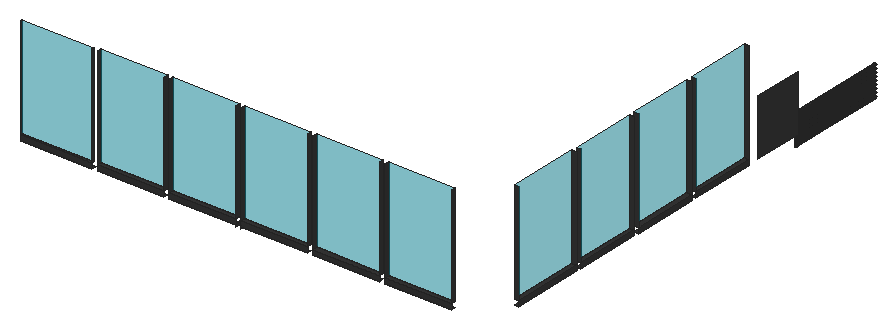
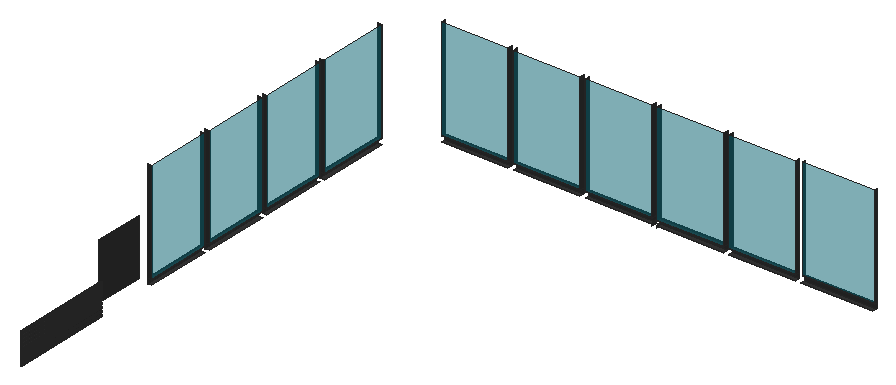
# SketchUp Ruby script. Lengths in inches.
U = 1.inch
M = Sketchup.active_model
def pt(a) = Geom::Point3d.new(a.map { |v| v * U })
def face(e, loops, mat)
  f = e.add_face(loops[0].map { |a| pt(a) })
  loops[1..].each { |l| e.add_face(l.map { |a| pt(a) }).erase! }
  f.material = f.back_material = mat if mat
  f
end
# faces: each face lists its corners as indices into pts; further lists are holes
def faces(e, pts, list, mat = nil) = list.each { |f| face(e, (f[0].is_a?(Array) ? f : [f]).map { |l| l.map { |i| pts[i] } }, mat) }
# xy, xz, yz: faces in a plane at the given z, y or x. An outline is a flat list of corners, or four numbers for a rectangle; further outlines are holes
def ring(l) = l.size == 4 ? [[l[0], l[1]], [l[2], l[1]], [l[2], l[3]], [l[0], l[3]]] : l.each_slice(2).to_a
def flat(e, list, mat, &to3) = list.each { |f| face(e, (f[0].is_a?(Array) ? f : [f]).map { |l| ring(l).map { |u, v| to3.(u, v) } }, mat) }
def xy(e, z, list, mat = nil) = flat(e, list, mat) { |x, y| [x, y, z] }
def xz(e, y, list, mat = nil) = flat(e, list, mat) { |x, z| [x, y, z] }
def yz(e, x, list, mat = nil) = flat(e, list, mat) { |y, z| [x, y, z] }
def lines(e, pts, list) = list.each { |a, b| e.add_line(pt(pts[a]), pt(pts[b])) }
# prism: a flat outline (further loops are holes) pulled along v
def prism(e, loops, v, mat = nil)
  f = face(e, loops, mat); d = Geom::Vector3d.new(v.map { |x| x * U })
  f.pushpull(f.normal.samedirection?(d) ? d.length : -d.length)
end
def box(e, o, s, mat = nil) = prism(e, [[o, [o[0] + s[0], o[1], o[2]], [o[0] + s[0], o[1] + s[1], o[2]], [o[0], o[1] + s[1], o[2]]]], [0, 0, s[2]], mat)
def at(x, y, z, deg = 0) = Geom::Transformation.translation(pt([x, y, z])) * Geom::Transformation.rotation(ORIGIN, Z_AXIS, deg.degrees)
def axes(o, x, y, z) = Geom::Transformation.new([*x, 0, *y, 0, *z, 0, *pt(o).to_a, 1])
def part(name) = M.definitions.add(name)
# library, detail: a bought-in or finely detailed component or shape, given as its bounding box
def library(name, o, s) = part(name).tap { |d| box(d.entities, o, s) }
def detail(e, o, s) = box(e.add_group.entities, o, s)
def put(e, d, t, mat = nil) = e.add_instance(d, t).tap { |i| i.material = mat if mat }
def group(e, t, mat = nil) = e.add_group.tap { |g| g.transformation = t; g.material = mat if mat }.entities
root = M.entities
M.materials.add("[0135_DarkGray]1").color = [53, 53, 53]
M.materials.add("[Translucent Glass Blue]1").color = [1, 149, 171]
M.materials["[Translucent Glass Blue]1"].alpha = 0.5
xy(root,442.86,[[1035.97,1165.35,1036.3125,1278.6875]],"[0135_DarkGray]1")
xy(root,445.46,[[1035.96,1165.35,1036.3,1278.6875]],"[0135_DarkGray]1")
xy(root,446.99,[[1035.97,1165.35,1036.3125,1278.6875]],"[0135_DarkGray]1")
xy(root,450.375,[[497.69,732.5625,579.69,737.5625],[585.69,732.5625,661.69,737.5625],[667.69,732.5625,743.69,737.5625],[749.69,732.5625,825.69,737.5625],[831.69,732.5625,907.69,737.5625],
  [913.69,732.5625,989.69,737.5625],[1028.13,774.6875,1033.13,856.6875],[1028.13,862.6875,1033.13,938.6875],[1028.13,944.6875,1033.13,1020.6875],[1028.13,1026.6875,1033.13,1102.6875]],"[0135_DarkGray]1")
xy(root,451.125,[[1035.97,1165.35,1036.3125,1278.6875]],"[0135_DarkGray]1")
xy(root,453.73,[[1035.96,1165.35,1036.3,1278.6875]],"[0135_DarkGray]1")
xy(root,455.26,[[1035.97,1165.35,1036.3125,1278.6875]],"[0135_DarkGray]1")
xy(root,456.375,[[497.69,732.5625,579.69,734.5625],[585.69,732.5625,661.69,737.5625],[667.69,732.5625,743.69,737.5625],[749.69,732.5625,825.69,737.5625],[831.69,732.5625,907.69,737.5625],
  [913.69,732.5625,989.69,737.5625],[1028.13,774.6875,1033.13,856.6875],[1028.13,862.6875,1033.13,938.6875],[1028.13,944.6875,1033.13,1020.6875],[1028.13,1026.6875,1033.13,1102.6875]],"[0135_DarkGray]1")
xy(root,457.86,[[1035.96,1165.35,1036.3,1278.6875]],"[0135_DarkGray]1")
xy(root,459.39,[[1035.97,1165.35,1036.3125,1278.6875]],"[0135_DarkGray]1")
xy(root,467.66,[[1035.97,1165.35,1036.3125,1278.6875]],"[0135_DarkGray]1")
xy(root,470.26,[[1035.96,1165.35,1036.3,1278.6875]],"[0135_DarkGray]1")
xy(root,471.79,[[1035.97,1165.35,1036.3125,1278.6875]],"[0135_DarkGray]1")
xy(root,478.53,[[1035.96,1165.35,1036.3,1278.6875]],"[0135_DarkGray]1")
xz(root,732.5625,[[497.69,450.375,579.69,456.375],[585.69,450.375,661.69,456.375],[667.69,450.375,743.69,456.375],[749.69,450.375,825.69,456.375],[831.69,450.375,907.69,456.375],
  [913.69,450.375,989.69,456.375]],"[0135_DarkGray]1")
xz(root,734.5625,[[497.69,456.375,579.69,572.5]],"[Translucent Glass Blue]1")
xz(root,737.5625,[[585.69,456.375,661.69,572.5],[667.69,456.375,743.69,572.5],[749.69,456.375,825.69,572.5],[831.69,456.375,907.69,572.5],[913.69,456.375,989.69,572.5]],"[Translucent Glass Blue]1")
xz(root,774.6875,[[1028.13,456.375,1033.13,572.5]],"[0135_DarkGray]1")
xz(root,856.6875,[[1028.13,456.375,1033.13,572.5]],"[0135_DarkGray]1")
xz(root,862.6875,[[1028.13,456.375,1033.13,572.5]],"[0135_DarkGray]1")
xz(root,938.6875,[[1028.13,456.375,1033.13,572.5]],"[0135_DarkGray]1")
xz(root,944.6875,[[1028.13,456.375,1033.13,572.5]],"[0135_DarkGray]1")
xz(root,1020.6875,[[1028.13,456.375,1033.13,572.5]],"[0135_DarkGray]1")
xz(root,1026.6875,[[1028.13,456.375,1033.13,572.5]],"[0135_DarkGray]1")
xz(root,1102.6875,[[1028.13,456.375,1033.13,572.5]],"[0135_DarkGray]1")
yz(root,497.69,[[732.5625,456.375,734.5625,572.5]],"[0135_DarkGray]1")
yz(root,579.69,[[732.5625,456.375,734.5625,572.5]],"[0135_DarkGray]1")
yz(root,585.69,[[732.5625,456.375,737.5625,572.5]],"[0135_DarkGray]1")
yz(root,661.69,[[732.5625,456.375,737.5625,572.5]],"[0135_DarkGray]1")
yz(root,667.69,[[732.5625,456.375,737.5625,572.5]],"[0135_DarkGray]1")
yz(root,743.69,[[732.5625,448.5,737.5625,450.375],[732.5625,456.375,737.5625,456.77],[732.5625,456.77,737.5625,572.5]],"[0135_DarkGray]1")
yz(root,749.69,[[732.5625,448.5,737.5625,450.375],[732.5625,456.375,737.5625,456.77],[732.5625,456.77,737.5625,572.5]],"[0135_DarkGray]1")
yz(root,825.69,[[732.5625,456.375,737.5625,572.5]],"[0135_DarkGray]1")
yz(root,831.69,[[732.5625,456.375,737.5625,572.5]],"[0135_DarkGray]1")
yz(root,907.69,[[732.5625,456.375,737.5625,572.5]],"[0135_DarkGray]1")
yz(root,913.69,[[732.5625,456.375,737.5625,572.5]],"[0135_DarkGray]1")
yz(root,989.69,[[732.5625,456.375,737.5625,572.5]],"[0135_DarkGray]1")
yz(root,1028.13,[[774.6875,456.375,856.6875,572.5],[862.6875,456.375,938.6875,572.5],[944.6875,456.375,1020.6875,572.5],[1026.6875,456.375,1102.6875,572.5]],"[Translucent Glass Blue]1")
yz(root,1033.13,[[774.6875,450.375,856.6875,456.375],[862.6875,450.375,938.6875,456.375],[944.6875,450.375,1020.6875,456.375],[1026.6875,450.375,1102.6875,456.375]],"[0135_DarkGray]1")
yz(root,1034.83,[[1165.35,443.98,1278.6875,444.32],[1165.35,448.11,1278.6875,448.46],[1165.35,452.25,1278.6875,452.59],[1165.35,456.38,1278.6875,456.72],[1165.35,460.51,1278.6875,460.86],
  [1165.35,464.65,1278.6875,464.99],[1165.35,468.78,1278.6875,469.125],[1165.35,472.91,1278.6875,473.26],[1165.35,477.05,1278.6875,477.39]],"[0135_DarkGray]1")
yz(root,1038.13,[[1108.6875,456.375,1165.35,520.4375]],"[0135_DarkGray]1")
p = [[1035.64,1165.35,442.94],[1035.34,1165.35,443.11],[1035.34,1278.6875,443.11],[1035.64,1278.6875,442.94],[1035.97,1165.35,442.86],[1035.97,1278.6875,442.86],
  [1036.64,1165.35,442.95],[1036.3125,1165.35,442.86],[1036.3125,1278.6875,442.86],[1036.64,1278.6875,442.95],[1036.94,1165.35,443.12],[1036.94,1278.6875,443.12],
  [1035.1,1165.35,443.35],[1035.1,1278.6875,443.35],[1037.18,1165.35,443.37],[1037.18,1278.6875,443.37],[1034.93,1165.35,443.65],[1034.93,1278.6875,443.65],
  [1037.35,1165.35,443.66],[1037.35,1278.6875,443.66],[1034.83,1165.35,443.98],[1034.83,1278.6875,443.98],[1037.4375,1165.35,444],[1037.4375,1278.6875,444],
  [1037.44,1165.35,444.34],[1037.44,1278.6875,444.34],[1034.83,1165.35,444.32],[1034.92,1165.35,444.65],[1034.92,1278.6875,444.65],[1034.83,1278.6875,444.32],
  [1037.34,1165.35,444.67],[1037.34,1278.6875,444.67],[1035.09,1165.35,444.95],[1035.09,1278.6875,444.95],[1037.17,1165.35,444.96],[1037.17,1278.6875,444.96],
  [1035.33,1165.35,445.2],[1035.33,1278.6875,445.2],[1036.93,1165.35,445.21],[1036.93,1278.6875,445.21],[1035.625,1165.35,445.37],[1035.625,1278.6875,445.37],
  [1036.63,1165.35,445.375],[1036.63,1278.6875,445.375],[1035.96,1165.35,445.46],[1035.96,1278.6875,445.46],[1036.3,1165.35,445.46],[1036.3,1278.6875,445.46],
  [1035.97,1165.35,446.99],[1035.64,1165.35,447.08],[1035.64,1278.6875,447.08],[1035.97,1278.6875,446.99],[1036.64,1165.35,447.08],[1036.3125,1165.35,446.99],
  [1036.3125,1278.6875,446.99],[1036.64,1278.6875,447.08],[1035.34,1165.35,447.25],[1035.34,1278.6875,447.25],[1036.94,1165.35,447.26],[1036.94,1278.6875,447.26],
  [1035.1,1165.35,447.49],[1035.1,1278.6875,447.49],[1037.18,1165.35,447.5],[1037.18,1278.6875,447.5],[1034.93,1165.35,447.78],[1034.93,1278.6875,447.78],
  [1037.35,1165.35,447.8],[1037.35,1278.6875,447.8],[1034.83,1165.35,448.11],[1034.83,1278.6875,448.11],[1037.4375,1165.35,448.13],[1037.4375,1278.6875,448.13],
  [1037.44,1165.35,448.47],[1037.44,1278.6875,448.47],[1034.83,1165.35,448.46],[1034.92,1165.35,448.79],[1034.92,1278.6875,448.79],[1034.83,1278.6875,448.46],
  [1037.34,1165.35,448.8],[1037.34,1278.6875,448.8],[1035.09,1165.35,449.09],[1035.09,1278.6875,449.09],[1037.17,1165.35,449.1],[1037.17,1278.6875,449.1],
  [1035.33,1165.35,449.33],[1035.33,1278.6875,449.33],[1036.93,1165.35,449.34],[1036.93,1278.6875,449.34],[1035.625,1165.35,449.5],[1035.625,1278.6875,449.5],
  [1036.63,1165.35,449.51],[1036.63,1278.6875,449.51],[1035.96,1165.35,449.59],[1035.96,1278.6875,449.59],[1036.3,1165.35,449.6],[1036.3,1278.6875,449.6],
  [1035.97,1165.35,451.125],[1035.64,1165.35,451.21],[1035.64,1278.6875,451.21],[1035.97,1278.6875,451.125],[1036.64,1165.35,451.22],[1036.3125,1165.35,451.125],
  [1036.3125,1278.6875,451.125],[1036.64,1278.6875,451.22],[1035.34,1165.35,451.38],[1035.34,1278.6875,451.38],[1036.94,1165.35,451.39],[1036.94,1278.6875,451.39],
  [1035.1,1165.35,451.62],[1035.1,1278.6875,451.62],[1037.18,1165.35,451.63],[1037.18,1278.6875,451.63],[1034.93,1165.35,451.92],[1034.93,1278.6875,451.92],
  [1037.35,1165.35,451.93],[1037.35,1278.6875,451.93],[1034.83,1165.35,452.25],[1034.83,1278.6875,452.25],[1037.4375,1165.35,452.26],[1037.4375,1278.6875,452.26],
  [1037.44,1165.35,452.6],[1037.44,1278.6875,452.6],[1034.83,1165.35,452.59],[1034.92,1165.35,452.92],[1034.92,1278.6875,452.92],[1034.83,1278.6875,452.59],
  [1037.34,1165.35,452.94],[1037.34,1278.6875,452.94],[1035.09,1165.35,453.22],[1035.09,1278.6875,453.22],[1037.17,1165.35,453.23],[1037.17,1278.6875,453.23],
  [1035.33,1165.35,453.46],[1035.33,1278.6875,453.46],[1036.93,1165.35,453.47],[1036.93,1278.6875,453.47],[1035.625,1165.35,453.64],[1035.625,1278.6875,453.64],
  [1036.63,1165.35,453.64],[1036.63,1278.6875,453.64],[1035.96,1165.35,453.73],[1035.96,1278.6875,453.73],[1036.3,1165.35,453.73],[1036.3,1278.6875,453.73],
  [1035.64,1165.35,455.34],[1035.34,1165.35,455.51],[1035.34,1278.6875,455.51],[1035.64,1278.6875,455.34],[1035.97,1165.35,455.26],[1035.97,1278.6875,455.26],
  [1036.64,1165.35,455.35],[1036.3125,1165.35,455.26],[1036.3125,1278.6875,455.26],[1036.64,1278.6875,455.35],[1036.94,1165.35,455.52],[1036.94,1278.6875,455.52],
  [1035.1,1165.35,455.75],[1035.1,1278.6875,455.75],[1037.18,1165.35,455.77],[1037.18,1278.6875,455.77],[1034.93,1165.35,456.05],[1034.93,1278.6875,456.05],
  [1037.35,1165.35,456.0625],[1037.35,1278.6875,456.0625],[1034.83,1165.35,456.38],[1034.83,1278.6875,456.38],[1037.4375,1165.35,456.4],[1037.4375,1278.6875,456.4],
  [1037.44,1165.35,456.74],[1037.44,1278.6875,456.74],[1034.83,1165.35,456.72],[1034.92,1165.35,457.05],[1034.92,1278.6875,457.05],[1034.83,1278.6875,456.72],
  [1037.34,1165.35,457.07],[1037.34,1278.6875,457.07],[1035.09,1165.35,457.35],[1035.09,1278.6875,457.35],[1037.17,1165.35,457.36],[1037.17,1278.6875,457.36],
  [1035.33,1165.35,457.6],[1035.33,1278.6875,457.6],[1036.93,1165.35,457.61],[1036.93,1278.6875,457.61],[1035.625,1165.35,457.77],[1035.625,1278.6875,457.77],
  [1036.63,1165.35,457.77],[1036.63,1278.6875,457.77],[1035.96,1165.35,457.86],[1035.96,1278.6875,457.86],[1036.3,1165.35,457.86],[1036.3,1278.6875,457.86],
  [1035.97,1165.35,459.39],[1035.64,1165.35,459.48],[1035.64,1278.6875,459.48],[1035.97,1278.6875,459.39],[1036.64,1165.35,459.48],[1036.3125,1165.35,459.39],
  [1036.3125,1278.6875,459.39],[1036.64,1278.6875,459.48],[1035.34,1165.35,459.65],[1035.34,1278.6875,459.65],[1036.94,1165.35,459.66],[1036.94,1278.6875,459.66],
  [1035.1,1165.35,459.89],[1035.1,1278.6875,459.89],[1037.18,1165.35,459.9],[1037.18,1278.6875,459.9],[1034.93,1165.35,460.18],[1034.93,1278.6875,460.18],
  [1037.35,1165.35,460.2],[1037.35,1278.6875,460.2],[1034.83,1165.35,460.51],[1034.83,1278.6875,460.51],[1037.4375,1165.35,460.53],[1037.4375,1278.6875,460.53],
  [1037.44,1165.35,460.87],[1037.44,1278.6875,460.87],[1034.83,1165.35,460.86],[1034.92,1165.35,461.1875],[1034.92,1278.6875,461.1875],[1034.83,1278.6875,460.86],
  [1037.34,1165.35,461.2],[1037.34,1278.6875,461.2],[1035.09,1165.35,461.49],[1035.09,1278.6875,461.49],[1037.17,1165.35,461.5],[1037.17,1278.6875,461.5],
  [1035.33,1165.35,461.73],[1035.33,1278.6875,461.73],[1036.93,1165.35,461.74],[1036.93,1278.6875,461.74],[1035.625,1165.35,461.9],[1035.625,1278.6875,461.9],
  [1036.63,1165.35,461.91],[1036.63,1278.6875,461.91],[1035.96,1165.35,461.99],[1035.96,1278.6875,461.99],[1036.3,1165.35,462],[1036.3,1278.6875,462],
  [1035.97,1165.35,463.52],[1035.64,1165.35,463.61],[1035.64,1278.6875,463.61],[1035.97,1278.6875,463.52],[1036.3125,1165.35,463.53],[1036.3125,1278.6875,463.53],
  [1036.64,1165.35,463.62],[1036.64,1278.6875,463.62],[1035.34,1165.35,463.78],[1035.34,1278.6875,463.78],[1036.94,1165.35,463.79],[1036.94,1278.6875,463.79],
  [1035.1,1165.35,464.02],[1035.1,1278.6875,464.02],[1037.18,1165.35,464.03],[1037.18,1278.6875,464.03],[1034.93,1165.35,464.32],[1034.93,1278.6875,464.32],
  [1037.35,1165.35,464.33],[1037.35,1278.6875,464.33],[1034.83,1165.35,464.65],[1034.83,1278.6875,464.65],[1037.4375,1165.35,464.66],[1037.4375,1278.6875,464.66],
  [1037.44,1165.35,465],[1037.44,1278.6875,465],[1034.83,1165.35,464.99],[1034.92,1165.35,465.32],[1034.92,1278.6875,465.32],[1034.83,1278.6875,464.99],
  [1037.34,1165.35,465.34],[1037.34,1278.6875,465.34],[1035.09,1165.35,465.62],[1035.09,1278.6875,465.62],[1037.17,1165.35,465.63],[1037.17,1278.6875,465.63],
  [1035.33,1165.35,465.86],[1035.33,1278.6875,465.86],[1036.93,1165.35,465.87],[1036.93,1278.6875,465.87],[1035.625,1165.35,466.04],[1035.625,1278.6875,466.04],
  [1036.63,1165.35,466.04],[1036.63,1278.6875,466.04],[1035.96,1165.35,466.125],[1035.96,1278.6875,466.125],[1036.3,1165.35,466.13],[1036.3,1278.6875,466.13],
  [1035.64,1165.35,467.74],[1035.34,1165.35,467.91],[1035.34,1278.6875,467.91],[1035.64,1278.6875,467.74],[1035.97,1165.35,467.66],[1035.97,1278.6875,467.66],
  [1036.64,1165.35,467.75],[1036.3125,1165.35,467.66],[1036.3125,1278.6875,467.66],[1036.64,1278.6875,467.75],[1036.94,1165.35,467.92],[1036.94,1278.6875,467.92],
  [1035.1,1165.35,468.15],[1035.1,1278.6875,468.15],[1037.18,1165.35,468.17],[1037.18,1278.6875,468.17],[1034.93,1165.35,468.45],[1034.93,1278.6875,468.45],
  [1037.35,1165.35,468.46],[1037.35,1278.6875,468.46],[1034.83,1165.35,468.78],[1034.83,1278.6875,468.78],[1037.4375,1165.35,468.8],[1037.4375,1278.6875,468.8],
  [1037.44,1165.35,469.14],[1037.44,1278.6875,469.14],[1034.83,1165.35,469.125],[1034.92,1165.35,469.45],[1034.92,1278.6875,469.45],[1034.83,1278.6875,469.125],
  [1037.34,1165.35,469.47],[1037.34,1278.6875,469.47],[1035.09,1165.35,469.75],[1035.09,1278.6875,469.75],[1037.17,1165.35,469.76],[1037.17,1278.6875,469.76],
  [1035.33,1165.35,470],[1035.33,1278.6875,470],[1036.93,1165.35,470.01],[1036.93,1278.6875,470.01],[1035.625,1165.35,470.17],[1035.625,1278.6875,470.17],
  [1036.63,1165.35,470.17],[1036.63,1278.6875,470.17],[1035.96,1165.35,470.26],[1035.96,1278.6875,470.26],[1036.3,1165.35,470.26],[1036.3,1278.6875,470.26],
  [1035.97,1165.35,471.79],[1035.64,1165.35,471.88],[1035.64,1278.6875,471.88],[1035.97,1278.6875,471.79],[1036.64,1165.35,471.88],[1036.3125,1165.35,471.79],
  [1036.3125,1278.6875,471.79],[1036.64,1278.6875,471.88],[1035.34,1165.35,472.05],[1035.34,1278.6875,472.05],[1036.94,1165.35,472.06],[1036.94,1278.6875,472.06],
  [1035.1,1165.35,472.29],[1035.1,1278.6875,472.29],[1037.18,1165.35,472.3],[1037.18,1278.6875,472.3],[1034.93,1165.35,472.58],[1034.93,1278.6875,472.58],
  [1037.35,1165.35,472.6],[1037.35,1278.6875,472.6],[1034.83,1165.35,472.91],[1034.83,1278.6875,472.91],[1037.4375,1165.35,472.93],[1037.4375,1278.6875,472.93],
  [1037.44,1165.35,473.27],[1037.44,1278.6875,473.27],[1034.83,1165.35,473.26],[1034.92,1165.35,473.59],[1034.92,1278.6875,473.59],[1034.83,1278.6875,473.26],
  [1037.34,1165.35,473.6],[1037.34,1278.6875,473.6],[1035.09,1165.35,473.89],[1035.09,1278.6875,473.89],[1037.17,1165.35,473.9],[1037.17,1278.6875,473.9],
  [1035.33,1165.35,474.13],[1035.33,1278.6875,474.13],[1036.93,1165.35,474.14],[1036.93,1278.6875,474.14],[1035.625,1165.35,474.3],[1035.625,1278.6875,474.3],
  [1036.63,1165.35,474.31],[1036.63,1278.6875,474.31],[1035.96,1165.35,474.39],[1035.96,1278.6875,474.39],[1036.3,1165.35,474.4],[1036.3,1278.6875,474.4],
  [1035.97,1165.35,475.92],[1035.64,1165.35,476.01],[1035.64,1278.6875,476.01],[1035.97,1278.6875,475.92],[1036.3125,1165.35,475.93],[1036.3125,1278.6875,475.93],
  [1036.64,1165.35,476.02],[1036.64,1278.6875,476.02],[1035.34,1165.35,476.18],[1035.34,1278.6875,476.18],[1036.94,1165.35,476.1875],[1036.94,1278.6875,476.1875],
  [1035.1,1165.35,476.42],[1035.1,1278.6875,476.42],[1037.18,1165.35,476.43],[1037.18,1278.6875,476.43],[1034.93,1165.35,476.72],[1034.93,1278.6875,476.72],
  [1037.35,1165.35,476.73],[1037.35,1278.6875,476.73],[1034.83,1165.35,477.05],[1034.83,1278.6875,477.05],[1037.4375,1165.35,477.0625],[1037.4375,1278.6875,477.0625],
  [1037.44,1165.35,477.4],[1037.44,1278.6875,477.4],[1034.83,1165.35,477.39],[1034.92,1165.35,477.72],[1034.92,1278.6875,477.72],[1034.83,1278.6875,477.39],
  [1037.34,1165.35,477.74],[1037.34,1278.6875,477.74],[1035.09,1165.35,478.02],[1035.09,1278.6875,478.02],[1037.17,1165.35,478.03],[1037.17,1278.6875,478.03],
  [1035.33,1165.35,478.26],[1035.33,1278.6875,478.26],[1036.93,1165.35,478.27],[1036.93,1278.6875,478.27],[1035.625,1165.35,478.4375],[1035.625,1278.6875,478.4375],
  [1036.63,1165.35,478.44],[1036.63,1278.6875,478.44],[1035.96,1165.35,478.53],[1035.96,1278.6875,478.53],[1036.3,1165.35,478.53],[1036.3,1278.6875,478.53],
  [749.69,737.5625,452.63],[749.69,732.5625,452.63],[743.69,737.5625,452.63],[743.69,732.5625,452.63]]
faces(root,p,[[0,1,2,3],[4,0,3,5],[6,7,8,9],[10,6,9,11],[1,12,13,2],[14,10,11,15],[12,16,17,13],[18,14,15,19],
  [16,20,21,17],[22,18,19,23],[24,22,23,25],[26,27,28,29],[30,24,25,31],[27,32,33,28],[34,30,31,35],[32,36,37,33],
  [38,34,35,39],[36,40,41,37],[42,38,39,43],[40,44,45,41],[46,42,43,47],[48,49,50,51],[52,53,54,55],[49,56,57,50],
  [58,52,55,59],[56,60,61,57],[62,58,59,63],[60,64,65,61],[66,62,63,67],[64,68,69,65],[70,66,67,71],[72,70,71,73],
  [74,75,76,77],[78,72,73,79],[75,80,81,76],[82,78,79,83],[80,84,85,81],[86,82,83,87],[84,88,89,85],[90,86,87,91],
  [88,92,93,89],[94,90,91,95],[92,94,95,93],[96,97,98,99],[100,101,102,103],[97,104,105,98],[106,100,103,107],[104,108,109,105],
  [110,106,107,111],[108,112,113,109],[114,110,111,115],[112,116,117,113],[118,114,115,119],[120,118,119,121],[122,123,124,125],[126,120,121,127],
  [123,128,129,124],[130,126,127,131],[128,132,133,129],[134,130,131,135],[132,136,137,133],[138,134,135,139],[136,140,141,137],[142,138,139,143],
  [144,145,146,147],[148,144,147,149],[150,151,152,153],[154,150,153,155],[145,156,157,146],[158,154,155,159],[156,160,161,157],[162,158,159,163],
  [160,164,165,161],[166,162,163,167],[168,166,167,169],[170,171,172,173],[174,168,169,175],[171,176,177,172],[178,174,175,179],[176,180,181,177],
  [182,178,179,183],[180,184,185,181],[186,182,183,187],[184,188,189,185],[190,186,187,191],[192,193,194,195],[196,197,198,199],[193,200,201,194],
  [202,196,199,203],[200,204,205,201],[206,202,203,207],[204,208,209,205],[210,206,207,211],[208,212,213,209],[214,210,211,215],[216,214,215,217],
  [218,219,220,221],[222,216,217,223],[219,224,225,220],[226,222,223,227],[224,228,229,225],[230,226,227,231],[228,232,233,229],[234,230,231,235],
  [232,236,237,233],[238,234,235,239],[236,238,239,237],[240,241,242,243],[244,240,243,245],[246,244,245,247],[241,248,249,242],[250,246,247,251],
  [248,252,253,249],[254,250,251,255],[252,256,257,253],[258,254,255,259],[256,260,261,257],[262,258,259,263],[264,262,263,265],[266,267,268,269],
  [270,264,265,271],[267,272,273,268],[274,270,271,275],[272,276,277,273],[278,274,275,279],[276,280,281,277],[282,278,279,283],[280,284,285,281],
  [286,282,283,287],[284,286,287,285],[288,289,290,291],[292,288,291,293],[294,295,296,297],[298,294,297,299],[289,300,301,290],[302,298,299,303],
  [300,304,305,301],[306,302,303,307],[304,308,309,305],[310,306,307,311],[312,310,311,313],[314,315,316,317],[318,312,313,319],[315,320,321,316],
  [322,318,319,323],[320,324,325,321],[326,322,323,327],[324,328,329,325],[330,326,327,331],[328,332,333,329],[334,330,331,335],[336,337,338,339],
  [340,341,342,343],[337,344,345,338],[346,340,343,347],[344,348,349,345],[350,346,347,351],[348,352,353,349],[354,350,351,355],[352,356,357,353],
  [358,354,355,359],[360,358,359,361],[362,363,364,365],[366,360,361,367],[363,368,369,364],[370,366,367,371],[368,372,373,369],[374,370,371,375],
  [372,376,377,373],[378,374,375,379],[376,380,381,377],[382,378,379,383],[380,382,383,381],[384,385,386,387],[388,384,387,389],[390,388,389,391],
  [385,392,393,386],[394,390,391,395],[392,396,397,393],[398,394,395,399],[396,400,401,397],[402,398,399,403],[400,404,405,401],[406,402,403,407],
  [408,406,407,409],[410,411,412,413],[414,408,409,415],[411,416,417,412],[418,414,415,419],[416,420,421,417],[422,418,419,423],[420,424,425,421],
  [426,422,423,427],[424,428,429,425],[430,426,427,431]],"[0135_DarkGray]1")
lines(root,p,[[432,433],[434,435]])
